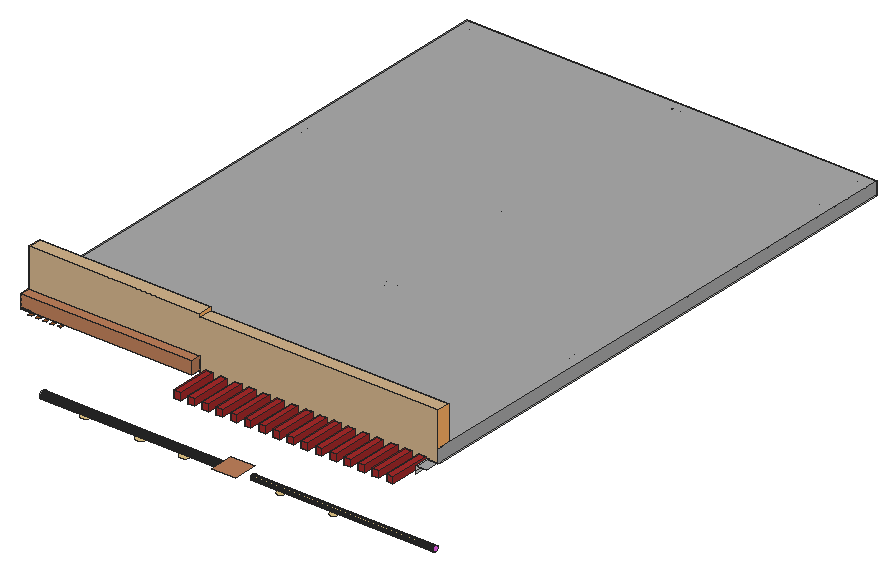
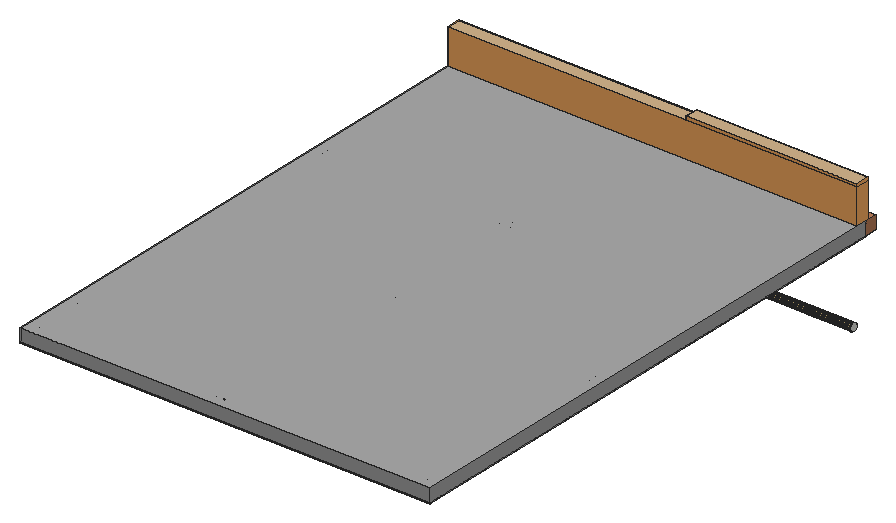
# SketchUp Ruby script. Lengths in inches.
U = 1.inch
M = Sketchup.active_model
def pt(a) = Geom::Point3d.new(a.map { |v| v * U })
def face(e, loops, mat)
  f = e.add_face(loops[0].map { |a| pt(a) })
  loops[1..].each { |l| e.add_face(l.map { |a| pt(a) }).erase! }
  f.material = f.back_material = mat if mat
  f
end
# faces: each face lists its corners as indices into pts; further lists are holes
def faces(e, pts, list, mat = nil) = list.each { |f| face(e, (f[0].is_a?(Array) ? f : [f]).map { |l| l.map { |i| pts[i] } }, mat) }
# xy, xz, yz: faces in a plane at the given z, y or x. An outline is a flat list of corners, or four numbers for a rectangle; further outlines are holes
def ring(l) = l.size == 4 ? [[l[0], l[1]], [l[2], l[1]], [l[2], l[3]], [l[0], l[3]]] : l.each_slice(2).to_a
def flat(e, list, mat, &to3) = list.each { |f| face(e, (f[0].is_a?(Array) ? f : [f]).map { |l| ring(l).map { |u, v| to3.(u, v) } }, mat) }
def xy(e, z, list, mat = nil) = flat(e, list, mat) { |x, y| [x, y, z] }
def xz(e, y, list, mat = nil) = flat(e, list, mat) { |x, z| [x, y, z] }
def yz(e, x, list, mat = nil) = flat(e, list, mat) { |y, z| [x, y, z] }
def lines(e, pts, list) = list.each { |a, b| e.add_line(pt(pts[a]), pt(pts[b])) }
# prism: a flat outline (further loops are holes) pulled along v
def prism(e, loops, v, mat = nil)
  f = face(e, loops, mat); d = Geom::Vector3d.new(v.map { |x| x * U })
  f.pushpull(f.normal.samedirection?(d) ? d.length : -d.length)
end
def box(e, o, s, mat = nil) = prism(e, [[o, [o[0] + s[0], o[1], o[2]], [o[0] + s[0], o[1] + s[1], o[2]], [o[0], o[1] + s[1], o[2]]]], [0, 0, s[2]], mat)
def at(x, y, z, deg = 0) = Geom::Transformation.translation(pt([x, y, z])) * Geom::Transformation.rotation(ORIGIN, Z_AXIS, deg.degrees)
def axes(o, x, y, z) = Geom::Transformation.new([*x, 0, *y, 0, *z, 0, *pt(o).to_a, 1])
def part(name) = M.definitions.add(name)
# library, detail: a bought-in or finely detailed component or shape, given as its bounding box
def library(name, o, s) = part(name).tap { |d| box(d.entities, o, s) }
def detail(e, o, s) = box(e.add_group.entities, o, s)
def put(e, d, t, mat = nil) = e.add_instance(d, t).tap { |i| i.material = mat if mat }
def group(e, t, mat = nil) = e.add_group.tap { |g| g.transformation = t; g.material = mat if mat }.entities
root = M.entities
M.materials.add("[0016_Tomato]").color = [255, 99, 71]
M.materials.add("[0018_Brown]").color = [165, 42, 42]
M.materials.add("[0035_Tan]").color = [210, 180, 140]
M.materials.add("[Color A03]").color = [255, 101, 101]
M.materials.add("[Color A08]1").color = [102, 0, 0]
M.materials.add("[Color B04]").color = [255, 101, 50]
M.materials.add("[Color C03]").color = [255, 178, 101]
M.materials.add("[Color K03]").color = [255, 101, 255]
M.materials.add("[Color M03]").color = [170, 170, 170]
M.materials.add("[Stone Brushed Khaki]").color = [226, 197, 133]
M.materials.add("[Wood Cherry Original]").color = [152, 86, 42]
M.materials.add("[Wood Veneer 02]").color = [190, 128, 91]
xy(root,161.89,[[133.81,324.96,181.81,330.96]])
xy(root,163.8125,[[263.46,39.6875,264.28,39.82,265.04,40.16,265.68,40.69,266.17,41.37,266.46,42.14,266.55,42.97,266.41,43.79,266.07,44.55,265.54,45.2,264.87,45.68,264.09,45.98,263.26,46.06,262.4375,45.92,261.68,45.58,261.04,45.05,260.55,44.38,260.26,43.6,260.17,42.77,260.31,41.95,260.65,41.19,261.18,40.55,261.85,40.0625,262.63,39.77]],"[Stone Brushed Khaki]")
xy(root,164.24,[[214.08,44.3,219.74,44.3,219.63,44.55,219.1,45.2,218.43,45.68,217.65,45.98,216.82,46.06,216,45.92,215.24,45.58,214.6,45.05,214.11,44.38]])
xy(root,164.24,[[217.02,39.6875,217.84,39.82,218.6,40.16,219.25,40.69,219.73,41.37,220.03,42.14,220.11,42.97,219.97,43.79,219.74,44.3,214.08,44.3,213.82,43.6,213.74,42.77,213.87,41.95,214.21,41.19,214.74,40.55,215.42,40.0625,216.19,39.77]],"[Stone Brushed Khaki]")
xy(root,164.88,[[129.19,42.4,137.7,42.4,137.67,42.6,137.24,43.66,136.99,43.99,129.91,43.99,129.66,43.66,129.22,42.6],[129.91,43.99,136.99,43.99,136.54,44.56,135.64,45.26,134.58,45.7,133.45,45.85,132.3125,45.7,131.26,45.26,130.35,44.56]])
xy(root,164.88,[[133.45,37.09,134.58,37.24,135.64,37.68,136.54,38.375,137.24,39.28,137.67,40.34,137.82,41.47,137.7,42.4,129.19,42.4,129.07,41.47,129.22,40.34,129.66,39.28,130.35,38.375,131.26,37.68,132.3125,37.24]],"[Stone Brushed Khaki]")
xy(root,165.0625,[[94.51,37.09,95.64,37.24,96.7,37.68,97.6,38.375,98.3,39.28,98.74,40.34,98.89,41.47,98.74,42.6,98.3,43.66,97.6,44.56,96.7,45.26,95.64,45.7,94.51,45.85,93.375,45.7,92.32,45.26,91.41,44.56,90.72,43.66,90.28,42.6,90.13,41.47,90.28,40.34,90.72,39.28,91.41,38.375,92.32,37.68,93.375,37.24]],"[Stone Brushed Khaki]")
xy(root,165.67,[[42.13,41.03,50.77,41.03,50.82,41.47,50.67,42.6,50.24,43.66,49.54,44.56,48.64,45.26,48.39,45.36,44.5,45.36,44.26,45.26,43.35,44.56,42.66,43.66,42.22,42.6,42.07,41.47],[44.5,45.36,48.39,45.36,47.58,45.7,46.45,45.85,45.3125,45.7]])
xy(root,165.67,[[46.45,37.09,47.58,37.24,48.64,37.68,49.54,38.375,50.24,39.28,50.67,40.34,50.77,41.03,42.13,41.03,42.22,40.34,42.66,39.28,43.35,38.375,44.26,37.68,45.3125,37.24]],"[Stone Brushed Khaki]")
xy(root,173.4375,[[169.02,27,190.02,48]],"[Wood Veneer 02]")
xy(root,204,[[188.875,246.36,194.875,282.36],[75.75,324.96,111.75,330.96]])
xy(root,209.89,[[133.81,324.96,181.81,330.96]])
xy(root,224.8125,[[246.73,191.3125,252.73,192.3125],[272.86,191.3125,278.86,192.3125],[300.23,191.3125,306.23,192.3125]],"[Color A08]1")
xy(root,234.8125,[[294.16,33,296.91,36],[300.29,33,303.66,36],[307.04,33,310.41,36],[313.79,33,317.16,36],[320.54,33,323.91,36],
  [327.29,33,330.66,36],[334.04,33,337.41,36],[340.79,33,344.16,36],[347.13,33,351.25,36],[151.38,36,351.25,39]])
xy(root,236.72,[[156.66,0,162.6,36]],"[0016_Tomato]")
xy(root,236.72,[[169.16,0,175.1,36],[181.66,0,187.6,36],[194.16,0,200.1,36],[206.66,0,212.6,36],[219.16,0,225.1,36],
  [231.66,0,237.6,36],[244.16,0,250.1,36],[256.66,0,262.6,36],[269.16,0,275.1,36],[281.66,0,287.6,36],
  [294.16,0,300.1,36],[306.66,0,312.6,36],[319.16,0,325.1,36],[331.66,0,337.6,36],[344.16,0,350.1,36]],"[0018_Brown]")
xy(root,240,[[0.25,27,9.25,39],[0,39,0.25,324.375],[0.25,39,9.25,324.375],[9.25,39,9.25,324.375,185.625,324.375,185.625,198.3125,188.875,198.3125,188.875,192.3125,351.25,192.3125,351.25,39],[360.25,39,360.625,468.3125],
  [185.625,198.3125,188.875,324.375],[194.875,198.3125,351.25,200.1875],[0,324.375,0.25,519],[9.25,324.375,187.9375,324.96],[187.9375,324.375,188.875,324.96],
  [188.875,330.375,188.29,330.96,188.875,330.96],[9.25,330.96,187.9375,331.75],[187.9375,330.96,188.875,331.75],[9.25,331.75,187.9375,510],[187.9375,331.75,188.875,510],
  [360.25,468.3125,360.625,519],[9.25,510,9.25,519,0.25,519]])
xy(root,240,[[9.25,324.96,187.9375,330.96],[187.9375,324.96,187.9375,330.96,188.29,330.96,188.875,330.375,188.875,324.96],[188.875,330.375,188.29,330.96,188.875,330.96]],"[Color A03]")
xy(root,240,[[351.25,39,360.25,468.3125],[188.875,192.3125,351.25,198.3125],[188.875,198.3125,194.875,200.1875],[188.875,200.1875,194.875,324.375],[0.25,324.375,0.25,519,9.25,510,9.25,324.375],
  [188.875,324.375,188.875,330.375,194.875,324.375],[194.875,324.375,188.875,330.375,188.875,510,194.875,510],[351.25,468.3125,360.25,468.3125,360.25,519,194.875,519,194.875,510,351.25,510],[9.25,510,194.875,519]],"[Color B04]")
xy(root,240,[[9.25,24,12.5,27],[15.75,24,19,27],[22.25,24,25.5,27],[28.75,24,32,27],[35.25,24,38.5,27]],"[Wood Cherry Original]")
xy(root,240.8125,[[0,27,9.25,39],[351.25,36,360.625,39],[0,39,360.625,519]])
xy(root,240.8125,[[351.25,24,360.25,36]],"[Color M03]")
xy(root,240.8125,[[9.25,27,151.38,39]],"[Wood Veneer 02]")
xy(root,240.9375,[[351.25,36,360.25,39]])
xy(root,241.375,[[0.25,27,9.25,39]])
xy(root,242.66,[[156.66,0,162.6,36],[169.16,0,175.1,36],[181.66,0,187.6,36],[194.16,0,200.1,36],[206.66,0,212.6,36],
  [219.16,0,225.1,36],[231.66,0,237.6,36],[244.16,0,250.1,36],[256.66,0,262.6,36],[269.16,0,275.1,36],
  [281.66,0,287.6,36],[294.16,0,300.1,36],[306.66,0,312.6,36],[319.16,0,325.1,36],[331.66,0,337.6,36],
  [344.16,0,350.1,36]],"[0018_Brown]")
xy(root,252,[[0.5,36,151.38,39],[0.5,39,151.38,48]])
xy(root,252,[[0,39,0.5,39,0.5,48,360.625,48,360.625,519,0,519]],"[Color M03]")
xy(root,252,[[0,27,151.38,27,151.38,36,0.5,36,0.5,39,0,39]],"[Wood Veneer 02]")
xy(root,282.71,[[151.38,36,360.625,48]],"[0035_Tan]")
xy(root,285.71,[[0.5,36,151.38,48]],"[0035_Tan]")
xz(root,0,[[156.66,236.72,162.6,242.66],[169.16,236.72,175.1,242.66],[181.66,236.72,187.6,242.66],[194.16,236.72,200.1,242.66],[206.66,236.72,212.6,242.66],
  [219.16,236.72,225.1,242.66],[231.66,236.72,237.6,242.66],[244.16,236.72,250.1,242.66],[256.66,236.72,262.6,242.66],[269.16,236.72,275.1,242.66],
  [281.66,236.72,287.6,242.66],[294.16,236.72,300.1,242.66],[306.66,236.72,312.6,242.66],[319.16,236.72,325.1,242.66],[331.66,236.72,337.6,242.66],
  [344.16,236.72,350.1,242.66]],"[0018_Brown]")
xz(root,27,[[0.25,240,9.25,240.8125],[0,240.8125,0.25,240.8125,0.25,241.375,9.25,241.375,9.25,240.8125,151.38,240.8125,151.38,252,0,252],[0.25,240.8125,9.25,241.375]],"[Wood Veneer 02]")
xz(root,36,[[294.16,234.8125,344.16,236.72],[344.16,234.8125,347.13,236.72],[347.13,234.8125,351.25,236.72],[156.66,236.72,162.6,242.66],[169.16,236.72,175.1,242.66],
  [181.66,236.72,187.6,242.66],[194.16,236.72,200.1,242.66],[206.66,236.72,212.6,242.66],[219.16,236.72,225.1,242.66],[231.66,236.72,237.6,242.66],
  [244.16,236.72,250.1,242.66],[256.66,236.72,262.6,242.66],[269.16,236.72,275.1,242.66],[281.66,236.72,287.6,242.66],[294.16,236.72,300.1,242.66],
  [306.66,236.72,312.6,242.66],[319.16,236.72,325.1,242.66],[331.66,236.72,337.6,242.66],[344.16,236.72,350.1,242.66],[351.25,240.8125,360.25,240.9375]])
xz(root,36,[[[151.38,234.8125,294.16,234.8125,294.16,242.66,300.1,242.66,300.1,236.72,306.66,236.72,306.66,242.66,312.6,242.66,312.6,236.72,319.16,236.72,319.16,242.66,325.1,242.66,325.1,236.72,331.66,236.72,331.66,242.66,337.6,242.66,337.6,236.72,344.16,236.72,344.16,242.66,350.1,242.66,350.1,236.72,351.25,236.72,351.25,240.9375,360.25,240.9375,360.25,240.8125,360.625,240.8125,360.625,282.71,151.38,282.71,151.38,285.71,0.5,285.71,0.5,252,151.38,252],[281.66,236.72,287.6,242.66],[269.16,236.72,275.1,242.66],[256.66,236.72,262.6,242.66],[244.16,236.72,250.1,242.66],[231.66,236.72,237.6,242.66],[219.16,236.72,225.1,242.66],[206.66,236.72,212.6,242.66],[194.16,236.72,200.1,242.66],[181.66,236.72,187.6,242.66],[169.16,236.72,175.1,242.66],[156.66,236.72,162.6,242.66]]],"[0035_Tan]")
xz(root,39,[[151.38,234.8125,351.25,240],[0,240,0.25,240.8125],[0.25,240,9.25,240.8125],[9.25,240,151.38,240.8125],[151.38,240,351.25,240.8125],
  [351.25,240,360.25,240.8125],[360.25,240,360.625,240.8125],[0,240.8125,0,252,151.38,252,151.38,240.8125,9.25,240.8125,9.25,241.375,0.25,241.375,0.25,240.8125],[0.25,240.8125,9.25,241.375],[351.25,240.8125,360.25,240.9375]])
xz(root,48,[[0.5,252,360.625,282.71],[0.5,282.71,151.38,285.71]],"[Color C03]")
xz(root,510,[[187.9375,240,188.875,252]])
xz(root,519,[[0,240,360.625,240.8125],[0,240.8125,360.625,252]],"[Color M03]")
yz(root,0,[[39,240,519,240.8125],[39,240.8125,519,252]],"[Color M03]")
yz(root,0,[[27,240.8125,39,252]],"[Wood Veneer 02]")
yz(root,0.25,[[27,240,39,241.375]],"[Wood Veneer 02]")
yz(root,0.5,[[36,252,48,282.71],[36,282.71,48,285.71]],"[Color C03]")
yz(root,6.77,[[43.19,164.77,42.4,164.88,41.66,165.18,41.03,165.67,40.54,166.3,40.24,167.04,40.13,167.84,40.24,168.63,40.54,169.37,41.03,170,41.66,170.49,42.4,170.79,43.19,170.9,43.99,170.79,44.73,170.49,45.36,170,45.85,169.37,46.15,168.63,46.26,167.84,46.15,167.04,45.85,166.3,45.36,165.67,44.73,165.18,43.99,164.88]])
yz(root,9.25,[[27,240,39,240.8125],[27,240.8125,39,241.375]])
yz(root,133.81,[[324.96,161.89,330.96,209.89]])
yz(root,151.38,[[36,234.8125,39,240.8125],[36,240.8125,39,252]])
yz(root,151.38,[[36,282.71,48,285.71]],"[Color C03]")
yz(root,151.38,[[27,240.8125,36,252]],"[Wood Veneer 02]")
yz(root,156.66,[[0,236.72,36,242.66]],"[0018_Brown]")
yz(root,162.6,[[0,236.72,36,242.66]],"[0018_Brown]")
yz(root,169.02,[[43.19,164.77,43.99,164.88,44.73,165.18,45.36,165.67,45.85,166.3,46.15,167.04,46.26,167.84,46.15,168.63,45.85,169.37,45.36,170,44.73,170.49,43.99,170.79,43.19,170.9,42.4,170.79,41.66,170.49,41.03,170,40.54,169.37,40.24,168.63,40.13,167.84,40.24,167.04,40.54,166.3,41.03,165.67,41.66,165.18,42.4,164.88]])
yz(root,169.16,[[0,236.72,36,242.66]],"[0018_Brown]")
yz(root,175.1,[[0,236.72,36,242.66]],"[0018_Brown]")
yz(root,181.66,[[0,236.72,36,242.66]],"[0018_Brown]")
yz(root,181.81,[[324.96,161.89,330.96,209.89]])
yz(root,187.6,[[0,236.72,36,242.66]],"[0018_Brown]")
yz(root,194.16,[[0,236.72,36,242.66]],"[0018_Brown]")
yz(root,200.1,[[0,236.72,36,242.66]],"[0018_Brown]")
yz(root,206.66,[[0,236.72,36,242.66]],"[0018_Brown]")
yz(root,212.6,[[0,236.72,36,242.66]],"[0018_Brown]")
yz(root,219.16,[[0,236.72,36,242.66]],"[0018_Brown]")
yz(root,225.1,[[0,236.72,36,242.66]],"[0018_Brown]")
yz(root,231.66,[[0,236.72,36,242.66]],"[0018_Brown]")
yz(root,237.6,[[0,236.72,36,242.66]],"[0018_Brown]")
yz(root,244.16,[[0,236.72,36,242.66]],"[0018_Brown]")
yz(root,250.1,[[0,236.72,36,242.66]],"[0018_Brown]")
yz(root,256.66,[[0,236.72,36,242.66]],"[0018_Brown]")
yz(root,262.6,[[0,236.72,36,242.66]],"[0018_Brown]")
yz(root,269.16,[[0,236.72,36,242.66]],"[0018_Brown]")
yz(root,275.1,[[0,236.72,36,242.66]],"[0018_Brown]")
yz(root,281.66,[[0,236.72,36,242.66]],"[0018_Brown]")
yz(root,287.6,[[0,236.72,36,242.66]],"[0018_Brown]")
yz(root,294.16,[[0,236.72,36,242.66]],"[0018_Brown]")
yz(root,300.1,[[0,236.72,36,242.66]],"[0018_Brown]")
yz(root,306.66,[[0,236.72,36,242.66]],"[0018_Brown]")
yz(root,312.6,[[0,236.72,36,242.66]],"[0018_Brown]")
yz(root,319.16,[[0,236.72,36,242.66]],"[0018_Brown]")
yz(root,325.1,[[0,236.72,36,242.66]],"[0018_Brown]")
yz(root,331.66,[[0,236.72,36,242.66]],"[0018_Brown]")
yz(root,337.6,[[0,236.72,36,242.66]],"[0018_Brown]")
yz(root,344.16,[[0,236.72,36,242.66]],"[0018_Brown]")
yz(root,350.1,[[0,236.72,36,242.66]],"[0018_Brown]")
yz(root,351.25,[[24,234.8125,36,236.72],[36,234.8125,39,240.8125],[24,236.72,36,240.8125],[36,240.8125,39,240.9375]])
yz(root,351.25,[[45.4,163.94,45.96,164.02,46.49,164.24,46.94,164.58,47.29,165.04,47.51,165.5625,47.58,166.13,47.51,166.7,47.29,167.22,46.94,167.68,46.49,168.02,45.96,168.24,45.4,168.32,44.83,168.24,44.3,168.02,43.85,167.68,43.5,167.22,43.28,166.7,43.21,166.13,43.28,165.5625,43.5,165.04,43.85,164.58,44.3,164.24,44.83,164.02]],"[Color K03]")
yz(root,360.625,[[39,240,519,240.8125]])
yz(root,360.625,[[36,252,48,282.71]],"[Color C03]")
yz(root,360.625,[[36,240.8125,519,252]],"[Color M03]")
p = [[351.25,45.4,163.94],[351.25,44.83,164.02],[190.02,44.83,164.02],[190.02,45.4,163.94],[351.25,45.96,164.02],[190.02,45.96,164.02],
  [351.25,44.3,164.24],[219.74,44.3,164.24],[214.08,44.3,164.24],[190.02,44.3,164.24],[351.25,46.49,164.24],[190.02,46.49,164.24],
  [351.25,43.85,164.58],[190.02,43.85,164.58],[351.25,46.94,164.58],[190.02,46.94,164.58],[351.25,43.5,165.04],[190.02,43.5,165.04],
  [351.25,47.29,165.04],[190.02,47.29,165.04],[169.02,43.19,164.77],[169.02,42.4,164.88],[137.7,42.4,164.88],[129.19,42.4,164.88],
  [6.77,42.4,164.88],[6.77,43.19,164.77],[169.02,43.99,164.88],[6.77,43.99,164.88],[129.91,43.99,164.88],[136.99,43.99,164.88],
  [169.02,41.66,165.18],[6.77,41.66,165.18],[169.02,44.73,165.18],[6.77,44.73,165.18],[351.25,43.28,165.5625],[190.02,43.28,165.5625],
  [351.25,47.51,165.5625],[190.02,47.51,165.5625],[169.02,41.03,165.67],[50.77,41.03,165.67],[42.13,41.03,165.67],[6.77,41.03,165.67],
  [169.02,45.36,165.67],[6.77,45.36,165.67],[44.5,45.36,165.67],[48.39,45.36,165.67],[351.25,43.21,166.13],[190.02,43.21,166.13],
  [351.25,47.58,166.13],[190.02,47.58,166.13],[169.02,40.54,166.3],[6.77,40.54,166.3],[169.02,45.85,166.3],[6.77,45.85,166.3],
  [351.25,43.28,166.7],[190.02,43.28,166.7],[351.25,47.51,166.7],[190.02,47.51,166.7],[169.02,40.24,167.04],[6.77,40.24,167.04],
  [169.02,46.15,167.04],[6.77,46.15,167.04],[351.25,43.5,167.22],[190.02,43.5,167.22],[351.25,47.29,167.22],[190.02,47.29,167.22],
  [169.02,40.13,167.84],[6.77,40.13,167.84],[169.02,46.26,167.84],[6.77,46.26,167.84],[351.25,43.85,167.68],[190.02,43.85,167.68],
  [351.25,46.94,167.68],[190.02,46.94,167.68],[351.25,44.3,168.02],[190.02,44.3,168.02],[351.25,46.49,168.02],[190.02,46.49,168.02],
  [169.02,40.24,168.63],[6.77,40.24,168.63],[169.02,46.15,168.63],[6.77,46.15,168.63],[351.25,44.83,168.24],[190.02,44.83,168.24],
  [351.25,45.96,168.24],[190.02,45.96,168.24],[351.25,45.4,168.32],[190.02,45.4,168.32],[169.02,40.54,169.37],[6.77,40.54,169.37],
  [169.02,45.85,169.37],[6.77,45.85,169.37],[169.02,41.03,170],[6.77,41.03,170],[169.02,45.36,170],[6.77,45.36,170],
  [169.02,41.66,170.49],[6.77,41.66,170.49],[169.02,44.73,170.49],[6.77,44.73,170.49],[169.02,42.4,170.79],[6.77,42.4,170.79],
  [169.02,43.99,170.79],[6.77,43.99,170.79],[169.02,43.19,170.9],[6.77,43.19,170.9],[133.81,324.96,185.89],[157.81,324.96,185.89],
  [157.81,324.96,161.89],[181.81,324.96,185.89],[157.81,324.96,209.89],[188.875,192.3125,240],[188.875,192.3125,252],[351.25,192.3125,240],
  [351.25,192.3125,252],[194.875,510,240],[194.875,510,252],[194.875,198.3125,240],[194.875,198.3125,252],[351.25,198.3125,240],
  [351.25,198.3125,252],[351.25,510,240],[351.25,510,252],[9.25,510,240],[9.25,510,252],[185.625,198.3125,240],
  [185.625,198.3125,252],[185.625,324.375,240],[185.625,324.375,252],[351.25,468.3125,240],[351.25,468.3125,252],[9.25,324.375,240],
  [9.25,324.375,252],[9.25,331.75,240],[9.25,331.75,252]]
faces(root,p,[[0,1,2,3],[4,0,3,5],[1,6,7,8,9,2],[10,4,5,11],[6,12,13,9,8,7],[14,10,11,15],[12,16,17,13],[18,14,15,19],
  [20,21,22,23,24,25],[26,20,25,27,28,29],[21,30,31,24,23,22],[32,26,29,28,27,33],[16,34,35,17],[36,18,19,37],[30,38,39,40,41,31],[42,32,33,43,44,45],
  [34,46,47,35],[48,36,37,49],[38,50,51,41,40,39],[52,42,45,44,43,53],[46,54,55,47],[56,48,49,57],[50,58,59,51],[60,52,53,61],
  [54,62,63,55],[64,56,57,65],[58,66,67,59],[68,60,61,69],[62,70,71,63],[72,64,65,73],[70,74,75,71],[76,72,73,77],
  [66,78,79,67],[80,68,69,81],[74,82,83,75],[84,76,77,85],[82,86,87,83],[86,84,85,87],[78,88,89,79],[90,80,81,91],
  [88,92,93,89],[94,90,91,95],[92,96,97,93],[98,94,95,99],[96,100,101,97],[102,98,99,103],[100,104,105,101],[104,102,103,105]],"[Stone Brushed Khaki]")
lines(root,p,[[106,107],[107,108],[107,109],[110,107],[111,112],[113,114],[115,116],[117,118],[119,120],[121,122],[123,124],[125,126],
  [127,128],[129,130],[131,132],[133,134]])
